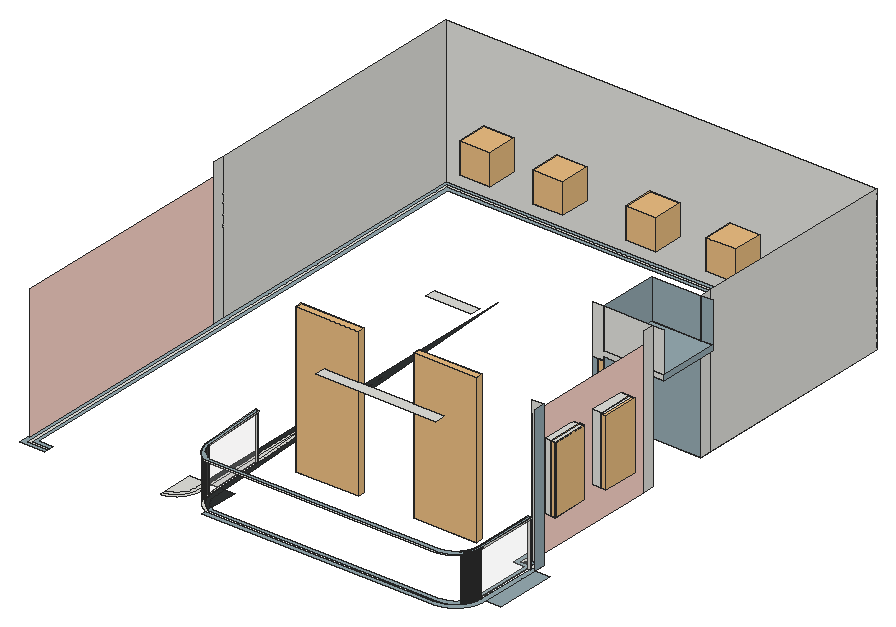
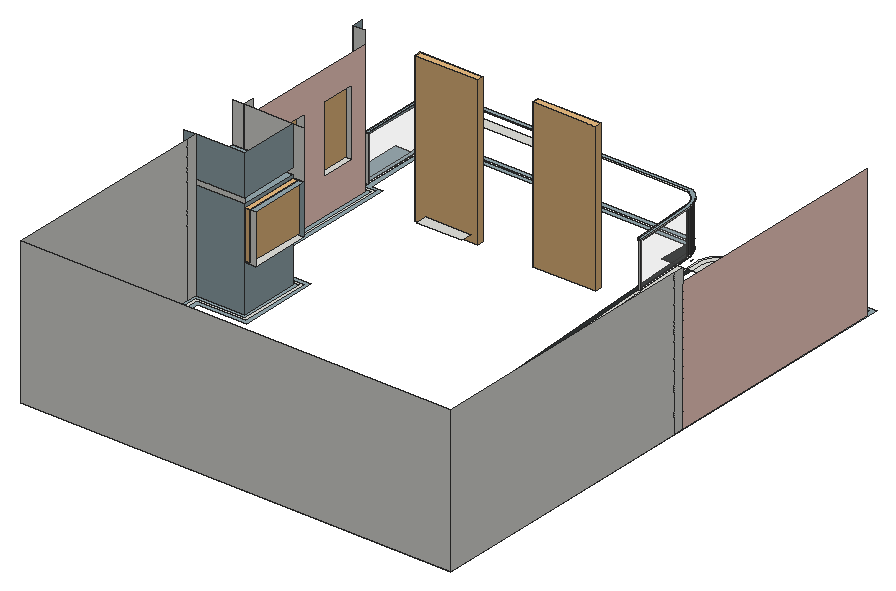
# SketchUp Ruby script. Lengths in inches.
U = 1.inch
M = Sketchup.active_model
def pt(a) = Geom::Point3d.new(a.map { |v| v * U })
def face(e, loops, mat)
  f = e.add_face(loops[0].map { |a| pt(a) })
  loops[1..].each { |l| e.add_face(l.map { |a| pt(a) }).erase! }
  f.material = f.back_material = mat if mat
  f
end
# faces: each face lists its corners as indices into pts; further lists are holes
def faces(e, pts, list, mat = nil) = list.each { |f| face(e, (f[0].is_a?(Array) ? f : [f]).map { |l| l.map { |i| pts[i] } }, mat) }
# xy, xz, yz: faces in a plane at the given z, y or x. An outline is a flat list of corners, or four numbers for a rectangle; further outlines are holes
def ring(l) = l.size == 4 ? [[l[0], l[1]], [l[2], l[1]], [l[2], l[3]], [l[0], l[3]]] : l.each_slice(2).to_a
def flat(e, list, mat, &to3) = list.each { |f| face(e, (f[0].is_a?(Array) ? f : [f]).map { |l| ring(l).map { |u, v| to3.(u, v) } }, mat) }
def xy(e, z, list, mat = nil) = flat(e, list, mat) { |x, y| [x, y, z] }
def xz(e, y, list, mat = nil) = flat(e, list, mat) { |x, z| [x, y, z] }
def yz(e, x, list, mat = nil) = flat(e, list, mat) { |y, z| [x, y, z] }
def lines(e, pts, list) = list.each { |a, b| e.add_line(pt(pts[a]), pt(pts[b])) }
# prism: a flat outline (further loops are holes) pulled along v
def prism(e, loops, v, mat = nil)
  f = face(e, loops, mat); d = Geom::Vector3d.new(v.map { |x| x * U })
  f.pushpull(f.normal.samedirection?(d) ? d.length : -d.length)
end
def box(e, o, s, mat = nil) = prism(e, [[o, [o[0] + s[0], o[1], o[2]], [o[0] + s[0], o[1] + s[1], o[2]], [o[0], o[1] + s[1], o[2]]]], [0, 0, s[2]], mat)
def at(x, y, z, deg = 0) = Geom::Transformation.translation(pt([x, y, z])) * Geom::Transformation.rotation(ORIGIN, Z_AXIS, deg.degrees)
def axes(o, x, y, z) = Geom::Transformation.new([*x, 0, *y, 0, *z, 0, *pt(o).to_a, 1])
def part(name) = M.definitions.add(name)
# library, detail: a bought-in or finely detailed component or shape, given as its bounding box
def library(name, o, s) = part(name).tap { |d| box(d.entities, o, s) }
def detail(e, o, s) = box(e.add_group.entities, o, s)
def put(e, d, t, mat = nil) = e.add_instance(d, t).tap { |i| i.material = mat if mat }
def group(e, t, mat = nil) = e.add_group.tap { |g| g.transformation = t; g.material = mat if mat }.entities
root = M.entities
M.materials.add("Generic").color = [150, 171, 178]
M.materials.add("Generic\#1").color = [47, 50, 50]
M.materials.add("Glass Thin Clear 001").color = [252, 250, 250]
M.materials["Glass Thin Clear 001"].alpha = 0.1
M.materials.add("[Color B01]").color = [255, 216, 204]
c1 = library("Curtains 003",[-24.98,-2.79,0.01],[49.96,5.58,117.31])
c2 = library("Window 46-05",[-17.86,-2.78,0],[35.72,4.26,58.96])
c3 = library("Window 46-06",[-34.91,-2.12,0],[69.82,4.27,59.06])
c4 = library("Omni Light",[-12,-12,-12],[24,24,24])
xy(root,257,[[13.326,45.171,29.81,45.171,29.81,46.928,15.083,46.928,15.083,460.197,347.352,460.197,347.352,295.928,308.352,295.928,308.352,238.197,347.352,238.197,347.352,118.197,356.352,118.197,356.352,114.0625,358.109,114.0625,358.109,119.954,349.109,119.954,349.109,239.954,310.109,239.954,310.109,294.171,349.109,294.171,349.109,461.954,13.326,461.954],[119.415,45.199,120.031,45.281,120.973,45.455,121.906,45.676,122.826,45.944,123.731,46.258,124.62,46.616,125.489,47.019,126.338,47.465,127.162,47.953,127.962,48.481,128.733,49.049,129.476,49.655,130.187,50.298,130.864,50.975,131.507,51.685,132.114,52.427,132.682,53.198,133.212,53.997,133.7,54.822,134.146,55.67,134.55,56.539,134.909,57.427,135.223,58.332,135.492,59.252,135.714,60.184,135.889,61.127,136.016,62.076,136.096,63.031,136.109,63.436,136.109,74.3125,134.352,74.3125,134.352,63.465,134.341,63.133,134.269,62.266,134.154,61.404,133.995,60.548,133.793,59.702,133.549,58.867,133.264,58.045,132.938,57.238,132.572,56.449,132.166,55.679,131.723,54.931,131.242,54.205,130.726,53.505,130.175,52.831,129.592,52.186,128.976,51.571,128.331,50.988,127.657,50.4375,126.956,49.922,126.23,49.442,125.481,48.999,124.711,48.594,123.922,48.229,123.115,47.903,122.293,47.618,121.457,47.375,120.611,47.174,119.755,47.016,119.415,46.971],[154.672,45.502,154.672,47.455,153.064,48.418,151.48,49.591,150.018,50.913,148.692,52.372,147.514,53.953,146.497,55.641,145.649,57.421,144.978,59.275,144.492,61.185,144.194,63.134,143.593,74.3125,141.834,74.3125,142.445,62.954,142.769,60.835,143.297,58.758,144.026,56.743,144.948,54.808,146.054,52.973,147.334,51.254,148.776,49.668,150.366,48.231,152.088,46.955,153.927,45.854],[119.415,46.971,119.755,47.016,120.611,47.174,121.457,47.375,122.293,47.618,123.115,47.903,123.922,48.229,124.711,48.594,125.481,48.999,126.23,49.442,126.956,49.922,127.657,50.4375,128.331,50.988,128.976,51.571,129.592,52.186,130.175,52.831,130.726,53.505,131.242,54.205,131.723,54.931,132.166,55.679,132.572,56.449,132.938,57.238,133.264,58.045,133.549,58.867,133.793,59.702,133.995,60.548,134.154,61.404,134.269,62.266,134.341,63.133,134.352,63.465,134.352,74.3125,131.151,74.3125,131.151,63.517,131.144,63.319,131.085,62.612,130.991,61.909,130.862,61.212,130.697,60.522,130.499,59.841,130.266,59.171,130,58.513,129.701,57.87,129.371,57.242,129.009,56.632,128.618,56.04,128.197,55.469,127.748,54.92,127.272,54.394,126.77,53.893,126.244,53.417,125.694,52.968,125.123,52.548,124.531,52.157,123.921,51.796,123.293,51.466,122.649,51.167,121.991,50.902,121.321,50.67,120.64,50.472,119.95,50.308,119.415,50.209],[119.415,50.209,119.95,50.308,120.64,50.472,121.321,50.67,121.991,50.902,122.649,51.167,123.293,51.466,123.921,51.796,124.531,52.157,125.123,52.548,125.694,52.968,126.244,53.417,126.77,53.893,127.272,54.394,127.748,54.92,128.197,55.469,128.618,56.04,129.009,56.632,129.371,57.242,129.701,57.87,130,58.513,130.266,59.171,130.499,59.841,130.697,60.522,130.862,61.212,130.991,61.909,131.085,62.612,131.144,63.319,131.151,63.517,131.151,74.3125,119.415,74.3125],
  [139.218,63.384,139.237,63.964,139.218,65.078],[134.352,74.3125,136.109,74.3125,136.109,180.704,139.695,114.0625,141.454,114.0625,134.352,246.036],[136.109,74.3125,141.834,74.3125,139.695,114.0625,136.109,180.704]])
xy(root,257,[[10.218,42.0625,29.81,42.0625,29.81,45.171,13.326,45.171,13.326,461.954,349.109,461.954,349.109,294.171,310.109,294.171,310.109,239.954,349.109,239.954,349.109,119.954,358.109,119.954,358.109,66.083,358.101,65.516,358.08,64.969,358.044,64.423,357.988,63.812,357.98,63.378,357.947,63.094,357.891,62.688,357.827,62.284,357.755,61.881,357.675,61.479,357.587,61.079,357.491,60.681,357.388,60.285,357.276,59.891,357.156,59.499,357.029,59.11,356.894,58.723,356.751,58.339,356.6,57.959,356.442,57.581,356.277,57.206,356.104,56.835,355.923,56.467,355.736,56.103,355.541,55.743,355.339,55.387,355.13,55.035,354.913,54.687,354.69,54.343,354.461,54.004,354.224,53.67,353.981,53.34,353.731,53.016,353.475,52.696,353.213,52.382,352.944,52.073,352.669,51.769,352.388,51.471,352.102,51.178,351.809,50.892,351.511,50.611,351.207,50.336,350.898,50.068,350.584,49.805,350.264,49.549,349.94,49.299,349.61,49.056,349.276,48.82,348.937,48.59,348.593,48.367,348.245,48.151,347.893,47.941,347.537,47.739,347.177,47.545,346.813,47.357,346.445,47.176,346.074,47.003,345.699,46.838,345.322,46.68,344.941,46.529,344.557,46.387,344.17,46.251,343.781,46.124,343.389,46.004,342.995,45.893,342.599,45.789,342.201,45.693,341.801,45.605,341.399,45.525,340.996,45.453,340.592,45.389,340.186,45.333,339.902,45.3,339.468,45.292,338.857,45.236,338.311,45.2,337.764,45.179,337.197,45.171,155.37,45.171,154.672,45.502,154.672,42.0625,337.222,42.0625,337.846,42.071,338.474,42.095,339.101,42.136,339.638,42.186,340.111,42.194,340.579,42.249,341.046,42.313,341.512,42.387,341.976,42.47,342.439,42.562,342.899,42.663,343.358,42.774,343.814,42.893,344.268,43.022,344.719,43.16,345.167,43.307,345.612,43.462,346.054,43.627,346.493,43.8,346.928,43.982,347.359,44.173,347.786,44.372,348.21,44.58,348.629,44.796,349.044,45.02,349.454,45.253,349.859,45.494,350.26,45.742,350.656,45.999,351.046,46.264,351.431,46.536,351.81,46.816,352.184,47.104,352.552,47.399,352.914,47.701,353.27,48.01,353.62,48.327,353.963,48.65,354.3,48.98,354.63,49.317,354.953,49.66,355.27,50.01,355.579,50.366,355.881,50.728,356.176,51.096,356.464,51.47,356.744,51.849,357.016,52.234,357.281,52.624,357.538,53.02,357.787,53.421,358.027,53.826,358.26,54.236,358.484,54.651,358.701,55.07,358.908,55.494,359.107,55.921,359.298,56.352,359.48,56.787,359.653,57.226,359.818,57.668,359.973,58.113,360.12,58.561,360.258,59.012,360.387,59.466,360.506,59.922,360.617,60.381,360.718,60.841,360.81,61.304,360.893,61.768,360.967,62.234,361.031,62.701,361.086,63.17,361.094,63.642,361.144,64.179,361.185,64.806,361.209,65.434,361.218,66.0625,361.218,123.0625,352.218,123.0625,352.218,243.0625,313.218,243.0625,313.218,291.0625,352.218,291.0625,352.218,465.0625,10.218,465.0625],[15.083,46.928,29.81,46.928,29.81,50.129,18.284,50.129,18.284,456.996,344.151,456.996,344.151,299.129,305.151,299.129,305.151,234.996,344.151,234.996,344.151,114.996,353.151,114.996,353.151,66.115,353.145,65.645,353.128,65.229,353.101,64.8125,353.034,64.082,353.028,63.713,352.986,63.413,352.938,63.106,352.883,62.801,352.823,62.496,352.756,62.193,352.683,61.891,352.604,61.59,352.519,61.292,352.429,60.995,352.332,60.699,352.23,60.406,352.121,60.115,352.007,59.826,351.887,59.54,351.762,59.256,351.631,58.974,351.494,58.695,351.351,58.419,351.204,58.146,351.05,57.876,350.892,57.609,350.728,57.345,350.559,57.085,350.385,56.828,350.205,56.574,350.021,56.324,349.831,56.078,349.637,55.836,349.438,55.597,349.234,55.363,349.026,55.132,348.813,54.906,348.596,54.684,348.374,54.467,348.148,54.254,347.917,54.046,347.683,53.842,347.445,53.643,347.202,53.449,346.956,53.259,346.706,53.075,346.453,52.896,346.196,52.721,345.935,52.552,345.671,52.388,345.404,52.23,345.134,52.076,344.861,51.929,344.585,51.786,344.306,51.65,344.024,51.518,343.74,51.393,343.454,51.273,343.165,51.159,342.874,51.05,342.581,50.948,342.286,50.851,341.988,50.761,341.69,50.676,341.389,50.597,341.087,50.524,340.784,50.458,340.479,50.397,340.174,50.342,339.867,50.294,339.567,50.253,339.198,50.246,338.468,50.179,338.051,50.152,337.635,50.135,337.165,50.129,156.484,50.129,156.266,50.232,154.844,51.084,154.672,51.212,154.672,47.455,154.755,47.405,155.765,46.928,337.186,46.928,337.718,46.935,338.219,46.954,338.719,46.987,339.372,47.047,339.784,47.054,339.964,47.075,340.335,47.127,340.705,47.185,341.073,47.251,341.441,47.324,341.806,47.404,342.171,47.492,342.533,47.587,342.893,47.689,343.251,47.799,343.607,47.915,343.961,48.039,344.312,48.169,344.66,48.307,345.005,48.452,345.348,48.603,345.6875,48.761,346.024,48.926,346.356,49.098,346.686,49.276,347.011,49.461,347.333,49.652,347.652,49.849,347.966,50.053,348.276,50.264,348.581,50.48,348.883,50.702,349.179,50.931,349.472,51.165,349.759,51.405,350.042,51.65,350.32,51.902,350.592,52.158,350.86,52.421,351.122,52.688,351.378,52.961,351.63,53.238,351.875,53.521,352.115,53.808,352.35,54.101,352.578,54.397,352.8,54.699,353.017,55.004,353.227,55.314,353.431,55.629,353.628,55.947,353.819,56.269,354.004,56.594,354.182,56.924,354.354,57.257,354.519,57.593,354.677,57.932,354.829,58.275,354.973,58.62,355.111,58.969,355.241,59.319,355.365,59.673,355.481,60.029,355.591,60.387,355.693,60.747,355.788,61.11,355.876,61.474,355.956,61.839,356.029,62.207,356.095,62.575,356.154,62.945,356.205,63.316,356.226,63.496,356.233,63.908,356.293,64.561,356.326,65.061,356.345,65.562,356.352,66.094,356.352,118.197,347.352,118.197,347.352,238.197,308.352,238.197,308.352,295.928,347.352,295.928,347.352,460.197,15.083,460.197],[361.218,66.0625,373.218,114.0625]],"Generic")
xy(root,257,[[154.672,47.455,154.672,51.212,153.511,52.071,152.281,53.183,151.166,54.41,150.175,55.74,149.319,57.16,148.606,58.657,148.042,60.216,147.633,61.823,147.383,63.462,146.799,74.3125,143.593,74.3125,144.194,63.134,144.492,61.185,144.978,59.275,145.649,57.421,146.497,55.641,147.514,53.953,148.692,52.372,150.018,50.913,151.48,49.591,153.064,48.418],[154.672,51.212,154.672,74.3125,146.799,74.3125,147.383,63.462,147.633,61.823,148.042,60.216,148.606,58.657,149.319,57.16,150.175,55.74,151.166,54.41,152.281,53.183,153.511,52.071],[131.151,74.3125,134.352,74.3125,134.352,246.036,141.454,114.0625,143.593,74.3125,146.799,74.3125,131.151,365.116]],"Generic\#1")
xy(root,285.591,[[352.218,135.565,361.218,163.627],[352.218,182.69,361.218,210.752]])
xy(root,293,[[155.245,44.615,153.664,45.363,151.779,46.492,150.013,47.8,148.383,49.274,146.905,50.9,145.592,52.662,144.458,54.544,143.512,56.528,142.765,58.595,142.223,60.724,141.891,62.897,139.108,114.619,141.981,114.619,144.748,63.191,145.037,61.296,145.51,59.438,146.162,57.635,146.987,55.905,147.976,54.263,149.121,52.726,150.411,51.308,151.833,50.022,153.373,48.881,155.018,47.896,155.889,47.484,337.182,47.484,337.704,47.491,338.19,47.51,338.675,47.541,339.342,47.603,339.746,47.61,339.894,47.627,340.254,47.677,340.613,47.733,340.97,47.797,341.327,47.868,341.682,47.946,342.035,48.031,342.386,48.124,342.736,48.223,343.083,48.329,343.429,48.442,343.772,48.562,344.112,48.689,344.45,48.822,344.786,48.962,345.118,49.109,345.447,49.263,345.774,49.423,346.097,49.589,346.416,49.762,346.732,49.942,347.045,50.127,347.353,50.319,347.658,50.517,347.959,50.721,348.256,50.931,348.548,51.146,348.836,51.368,349.12,51.595,349.399,51.828,349.673,52.066,349.942,52.31,350.207,52.559,350.466,52.814,350.721,53.073,350.97,53.338,351.214,53.607,351.452,53.881,351.685,54.16,351.912,54.444,352.134,54.732,352.35,55.024,352.559,55.321,352.763,55.622,352.961,55.927,353.153,56.235,353.339,56.548,353.518,56.864,353.691,57.183,353.857,57.506,354.017,57.833,354.171,58.162,354.318,58.494,354.458,58.83,354.591,59.168,354.718,59.508,354.838,59.851,354.951,60.197,355.057,60.544,355.157,60.894,355.249,61.245,355.334,61.599,355.412,61.953,355.483,62.31,355.547,62.668,355.604,63.026,355.653,63.386,355.67,63.534,355.677,63.938,355.739,64.605,355.77,65.09,355.79,65.576,355.796,66.098,355.796,114.619,358.665,114.619,358.665,66.079,358.657,65.501,358.635,64.94,358.599,64.38,358.544,63.781,358.536,63.341,358.499,63.024,358.441,62.607,358.376,62.192,358.302,61.778,358.22,61.365,358.129,60.954,358.031,60.545,357.924,60.138,357.809,59.734,357.686,59.331,357.555,58.932,357.417,58.535,357.27,58.14,357.115,57.749,356.953,57.361,356.783,56.976,356.605,56.595,356.42,56.217,356.227,55.843,356.027,55.474,355.82,55.108,355.605,54.746,355.383,54.389,355.154,54.036,354.918,53.6875,354.675,53.344,354.425,53.006,354.169,52.672,353.905,52.344,353.636,52.021,353.36,51.704,353.078,51.392,352.789,51.086,352.495,50.785,352.194,50.491,351.888,50.202,351.576,49.92,351.259,49.644,350.936,49.375,350.608,49.112,350.274,48.855,349.936,48.605,349.592,48.362,349.244,48.126,348.891,47.897,348.534,47.675,348.172,47.461,347.807,47.253,347.437,47.053,347.063,46.86,346.685,46.675,346.304,46.497,345.919,46.327,345.531,46.165,345.14,46.01,344.746,45.863,344.348,45.725,343.949,45.594,343.546,45.471,343.142,45.356,342.735,45.249,342.326,45.151,341.915,45.06,341.503,44.978,341.088,44.904,340.673,44.839,340.256,44.781,339.939,44.744,339.499,44.736,338.9,44.681,338.34,44.645,337.779,44.623,337.201,44.615]])
xy(root,294,[[155.245,44.615,337.201,44.615,337.779,44.623,338.34,44.645,338.9,44.681,339.499,44.736,339.939,44.744,340.256,44.781,340.673,44.839,341.088,44.904,341.503,44.978,341.915,45.06,342.326,45.151,342.735,45.249,343.142,45.356,343.546,45.471,343.949,45.594,344.348,45.725,344.746,45.863,345.14,46.01,345.531,46.165,345.919,46.327,346.304,46.497,346.685,46.675,347.063,46.86,347.437,47.053,347.807,47.253,348.172,47.461,348.534,47.675,348.891,47.897,349.244,48.126,349.592,48.362,349.936,48.605,350.274,48.855,350.608,49.112,350.936,49.375,351.259,49.644,351.576,49.92,351.888,50.202,352.194,50.491,352.495,50.785,352.789,51.086,353.078,51.392,353.36,51.704,353.636,52.021,353.905,52.344,354.169,52.672,354.425,53.006,354.675,53.344,354.918,53.6875,355.154,54.036,355.383,54.389,355.605,54.746,355.82,55.108,356.027,55.474,356.227,55.843,356.42,56.217,356.605,56.595,356.783,56.976,356.953,57.361,357.115,57.749,357.27,58.14,357.417,58.535,357.555,58.932,357.686,59.331,357.809,59.734,357.924,60.138,358.031,60.545,358.129,60.954,358.22,61.365,358.302,61.778,358.376,62.192,358.441,62.607,358.499,63.024,358.536,63.341,358.544,63.781,358.599,64.38,358.635,64.94,358.657,65.501,358.665,66.079,358.665,114.619,355.796,114.619,355.796,66.098,355.79,65.576,355.77,65.09,355.739,64.605,355.677,63.938,355.67,63.534,355.653,63.386,355.604,63.026,355.547,62.668,355.483,62.31,355.412,61.953,355.334,61.599,355.249,61.245,355.157,60.894,355.057,60.544,354.951,60.197,354.838,59.851,354.718,59.508,354.591,59.168,354.458,58.83,354.318,58.494,354.171,58.162,354.017,57.833,353.857,57.506,353.691,57.183,353.518,56.864,353.339,56.548,353.153,56.235,352.961,55.927,352.763,55.622,352.559,55.321,352.35,55.024,352.134,54.732,351.912,54.444,351.685,54.16,351.452,53.881,351.214,53.607,350.97,53.338,350.721,53.073,350.466,52.814,350.207,52.559,349.942,52.31,349.673,52.066,349.399,51.828,349.12,51.595,348.836,51.368,348.548,51.146,348.256,50.931,347.959,50.721,347.658,50.517,347.353,50.319,347.045,50.127,346.732,49.942,346.416,49.762,346.097,49.589,345.774,49.423,345.447,49.263,345.118,49.109,344.786,48.962,344.45,48.822,344.112,48.689,343.772,48.562,343.429,48.442,343.083,48.329,342.736,48.223,342.386,48.124,342.035,48.031,341.682,47.946,341.327,47.868,340.97,47.797,340.613,47.733,340.254,47.677,339.894,47.627,339.746,47.61,339.342,47.603,338.675,47.541,338.19,47.51,337.704,47.491,337.182,47.484,155.889,47.484,155.018,47.896,153.373,48.881,151.833,50.022,150.411,51.308,149.121,52.726,147.976,54.263,146.987,55.905,146.162,57.635,145.51,59.438,145.037,61.296,144.748,63.191,141.981,114.619,139.108,114.619,141.891,62.897,142.223,60.724,142.765,58.595,143.512,56.528,144.458,54.544,145.592,52.662,146.905,50.9,148.383,49.274,150.013,47.8,151.779,46.492,153.664,45.363]],"Generic")
xy(root,294.452,[[304.218,243.0625,313.218,291.0625]])
xy(root,333.326,[[304.218,243.0625,313.218,291.0625]],"Generic")
xy(root,335.818,[[313.218,243.0625,361.218,291.0625]],"Generic")
xy(root,336,[[187.218,114.0625,283.218,123.0625],[179.03,234.0625,215.03,243.0625]])
xy(root,338.859,[[352.218,135.565,361.218,163.627],[352.218,182.69,361.218,210.752]])
xy(root,340.246,[[313.218,243.0625,361.218,291.0625]],"Generic")
xz(root,114.0625,[[139.695,257,141.454,293],[356.352,257,358.109,293]])
xz(root,114.619,[[139.108,293,141.981,294],[355.796,293,358.665,294]])
xz(root,123.0625,[[352.218,257,361.218,372]])
xz(root,135.565,[[352.218,285.591,361.218,338.859]])
xz(root,163.627,[[352.218,285.591,361.218,338.859]])
xz(root,182.69,[[352.218,285.591,361.218,338.859]])
xz(root,210.752,[[352.218,285.591,361.218,338.859]])
xz(root,243.0625,[[304.218,333.326,304.218,372,313.218,372,313.218,340.246,352.218,340.246,352.218,335.818,313.218,335.818,313.218,333.326],[352.218,335.818,361.218,340.246],[313.218,340.246,352.218,372],[352.218,340.246,361.218,372]])
xz(root,243.0625,[[313.218,257,313.218,294.452,304.218,294.452,304.218,333.326,313.218,333.326,313.218,335.818,352.218,335.818,352.218,257]],"Generic")
xz(root,291.0625,[[304.218,294.452,313.218,333.326],[313.218,335.818,352.218,340.246],[352.218,335.818,361.218,340.246]])
xz(root,291.0625,[[313.218,257,352.218,335.818],[313.218,340.246,352.218,372],[352.218,340.246,361.218,372]],"Generic")
xz(root,465.0625,[[10.218,257,352.218,372]])
yz(root,10.218,[[234.0625,257,243.0625,372],[243.0625,257,465.0625,372]])
yz(root,10.218,[[51.0625,257,234.0625,362]],"[Color B01]")
yz(root,313.218,[[243.0625,257,291.0625,294.452],[243.0625,333.326,291.0625,335.818],[243.0625,340.246,291.0625,372]],"Generic")
yz(root,352.218,[[234.0625,257,243.0625,372],[291.0625,257,300.0625,372],[300.0625,257,465.0625,372]])
yz(root,352.218,[[[123.0625,257,234.0625,362],[182.69,285.591,210.752,338.859],[135.565,285.591,163.627,338.859]]],"[Color B01]")
yz(root,355.796,[[114.0625,293,114.619,294]])
yz(root,355.796,[[66.098,293,114.0625,294]],"Generic")
yz(root,355.977,[[66.097,293,111.931,294]])
yz(root,356.352,[[66.094,257,114.0625,293]],"Glass Thin Clear 001")
yz(root,358.109,[[66.083,257,114.0625,293]],"Glass Thin Clear 001")
yz(root,358.484,[[66.08,293,111.931,294]])
yz(root,358.665,[[66.079,293,114.619,294]])
yz(root,361.218,[[114.0625,257,123.0625,372],[243.0625,335.818,291.0625,340.246]],"Generic")
p = [[148.692,52.372,257],[147.514,53.953,257],[147.514,53.953,293],[148.692,52.372,293],[144.948,54.808,257],[146.054,52.973,257],
  [146.054,52.973,293],[144.948,54.808,293],[351.63,53.238,257],[351.378,52.961,257],[351.378,52.961,293],[351.63,53.238,293],
  [353.731,53.016,257],[353.981,53.34,257],[353.981,53.34,293],[353.731,53.016,293],[351.875,53.521,257],[351.875,53.521,293],
  [354.224,53.67,257],[354.224,53.67,293],[352.115,53.808,257],[352.115,53.808,293],[354.461,54.004,257],[354.461,54.004,293],
  [352.35,54.101,257],[352.35,54.101,293],[146.497,55.641,257],[146.497,55.641,293],[354.69,54.343,257],[354.69,54.343,293],
  [352.578,54.397,257],[352.578,54.397,293],[354.913,54.687,257],[354.913,54.687,293],[352.8,54.699,257],[352.8,54.699,293],
  [353.017,55.004,257],[353.017,55.004,293],[355.13,55.035,257],[355.13,55.035,293],[144.026,56.743,257],[144.026,56.743,293],
  [353.227,55.314,257],[353.227,55.314,293],[355.339,55.387,257],[355.339,55.387,293],[353.431,55.629,257],[353.431,55.629,293],
  [355.541,55.743,257],[355.541,55.743,293],[145.649,57.421,257],[145.649,57.421,293],[353.628,55.947,257],[353.628,55.947,293],
  [355.736,56.103,257],[355.736,56.103,293],[353.819,56.269,257],[353.819,56.269,293],[355.923,56.467,257],[355.923,56.467,293],
  [354.004,56.594,257],[354.004,56.594,293],[356.104,56.835,257],[356.104,56.835,293],[354.182,56.924,257],[354.182,56.924,293],
  [143.297,58.758,257],[143.297,58.758,293],[356.277,57.206,257],[356.277,57.206,293],[354.354,57.257,257],[354.354,57.257,293],
  [356.442,57.581,257],[356.442,57.581,293],[354.519,57.593,257],[354.519,57.593,293],[144.978,59.275,257],[144.978,59.275,293],
  [354.677,57.932,257],[354.677,57.932,293],[356.6,57.959,257],[356.6,57.959,293],[354.829,58.275,257],[354.829,58.275,293],
  [356.751,58.339,257],[356.751,58.339,293],[354.973,58.62,257],[354.973,58.62,293],[356.894,58.723,257],[356.894,58.723,293],
  [355.111,58.969,257],[355.111,58.969,293],[357.029,59.11,257],[357.029,59.11,293],[142.769,60.835,257],[142.769,60.835,293],
  [355.241,59.319,257],[355.241,59.319,293],[357.156,59.499,257],[357.156,59.499,293],[144.492,61.185,257],[144.492,61.185,293],
  [355.365,59.673,257],[355.365,59.673,293],[357.276,59.891,257],[357.276,59.891,293],[355.481,60.029,257],[355.481,60.029,293],
  [357.388,60.285,257],[357.388,60.285,293],[355.591,60.387,257],[355.591,60.387,293],[357.491,60.681,257],[357.491,60.681,293],
  [355.693,60.747,257],[355.693,60.747,293],[355.788,61.11,257],[355.788,61.11,293],[357.587,61.079,257],[357.587,61.079,293],
  [142.445,62.954,257],[142.445,62.954,293],[355.876,61.474,257],[355.876,61.474,293],[357.675,61.479,257],[357.675,61.479,293],
  [144.194,63.134,257],[144.194,63.134,293],[355.956,61.839,257],[355.956,61.839,293],[357.755,61.881,257],[357.755,61.881,293],
  [356.029,62.207,257],[356.029,62.207,293],[357.827,62.284,257],[357.827,62.284,293],[356.095,62.575,257],[356.095,62.575,293],
  [357.891,62.688,257],[357.891,62.688,293],[356.154,62.945,257],[356.154,62.945,293],[357.947,63.094,257],[357.947,63.094,293],
  [356.205,63.316,257],[356.205,63.316,293],[139.695,114.0625,257],[141.834,74.3125,257],[139.695,114.0625,293],[143.593,74.3125,257],
  [141.454,114.0625,257],[141.454,114.0625,293],[357.98,63.378,257],[357.98,63.378,293],[356.226,63.496,257],[356.226,63.496,293],
  [357.988,63.812,257],[357.988,63.812,293],[356.233,63.908,257],[356.233,63.908,293],[358.044,64.423,257],[358.044,64.423,293],
  [356.293,64.561,257],[356.293,64.561,293],[358.08,64.969,257],[358.08,64.969,293],[356.326,65.061,257],[356.326,65.061,293],
  [358.101,65.516,257],[358.101,65.516,293],[356.345,65.562,257],[356.345,65.562,293],[358.109,66.083,257],[358.109,66.083,293],
  [356.352,66.094,257],[356.352,66.094,293],[147.826,54.162,293],[147.826,54.162,294],[148.982,52.611,294],[148.982,52.611,293],
  [144.458,54.544,294],[144.458,54.544,293],[145.592,52.662,293],[145.592,52.662,294],[149.121,52.726,294],[149.121,52.726,293],
  [147.976,54.263,293],[147.976,54.263,294],[145.742,52.763,293],[145.742,52.763,294],[144.617,54.63,294],[144.617,54.63,293],
  [350.851,52.948,293],[350.851,52.948,294],[351.103,53.215,294],[351.103,53.215,293],[354.425,53.006,294],[354.425,53.006,293],
  [354.675,53.344,293],[354.675,53.344,294],[350.97,53.338,294],[350.97,53.338,293],[350.721,53.073,293],[350.721,53.073,294],
  [354.528,53.45,293],[354.528,53.45,294],[354.28,53.115,294],[354.28,53.115,293],[351.349,53.487,294],[351.349,53.487,293],
  [351.214,53.607,294],[351.214,53.607,293],[354.918,53.6875,293],[354.918,53.6875,294],[351.59,53.764,294],[351.59,53.764,293],
  [354.769,53.791,293],[354.769,53.791,294],[351.452,53.881,294],[351.452,53.881,293],[355.154,54.036,293],[355.154,54.036,294],
  [351.825,54.046,294],[351.825,54.046,293],[355.003,54.136,293],[355.003,54.136,294],[351.685,54.16,294],[351.685,54.16,293],
  [352.055,54.332,294],[352.055,54.332,293],[355.383,54.389,293],[355.383,54.389,294],[355.23,54.486,293],[355.23,54.486,294],
  [146.827,55.819,293],[146.827,55.819,294],[351.912,54.444,294],[351.912,54.444,293],[146.987,55.905,293],[146.987,55.905,294],
  [352.278,54.623,294],[352.278,54.623,293],[352.134,54.732,294],[352.134,54.732,293],[355.605,54.746,293],[355.605,54.746,294],
  [143.512,56.528,294],[143.512,56.528,293],[355.45,54.84,293],[355.45,54.84,294],[143.679,56.598,294],[143.679,56.598,293],
  [352.496,54.918,294],[352.496,54.918,293],[352.35,55.024,294],[352.35,55.024,293],[355.82,55.108,293],[355.82,55.108,294],
  [355.663,55.199,293],[355.663,55.199,294],[352.708,55.218,294],[352.708,55.218,293],[352.559,55.321,294],[352.559,55.321,293],
  [356.027,55.474,293],[356.027,55.474,294],[352.914,55.522,294],[352.914,55.522,293],[355.869,55.561,293],[355.869,55.561,294],
  [352.763,55.622,294],[352.763,55.622,293],[353.114,55.83,294],[353.114,55.83,293],[356.227,55.843,293],[356.227,55.843,294],
  [352.961,55.927,294],[352.961,55.927,293],[356.067,55.928,293],[356.067,55.928,294],[145.995,57.566,293],[145.995,57.566,294],
  [353.308,56.141,294],[353.308,56.141,293],[356.42,56.217,293],[356.42,56.217,294],[146.162,57.635,293],[146.162,57.635,294],
  [353.153,56.235,294],[353.153,56.235,293],[356.258,56.299,293],[356.258,56.299,294],[353.495,56.457,294],[353.495,56.457,293],
  [353.339,56.548,294],[353.339,56.548,293],[356.605,56.595,293],[356.605,56.595,294],[356.442,56.673,293],[356.442,56.673,294],
  [142.765,58.595,294],[142.765,58.595,293],[353.518,56.864,294],[353.518,56.864,293],[353.676,56.776,294],[353.676,56.776,293],
  [142.938,58.648,294],[142.938,58.648,293],[356.783,56.976,293],[356.783,56.976,294],[356.618,57.051,293],[356.618,57.051,294],
  [353.851,57.099,294],[353.851,57.099,293],[353.691,57.183,294],[353.691,57.183,293],[356.953,57.361,293],[356.953,57.361,294],
  [354.019,57.425,294],[354.019,57.425,293],[356.787,57.433,293],[356.787,57.433,294],[353.857,57.506,294],[353.857,57.506,293],
  [354.181,57.755,294],[354.181,57.755,293],[356.948,57.817,293],[356.948,57.817,294],[357.115,57.749,293],[357.115,57.749,294],
  [354.017,57.833,294],[354.017,57.833,293],[145.337,59.385,293],[145.337,59.385,294],[145.51,59.438,293],[145.51,59.438,294],
  [357.27,58.14,293],[357.27,58.14,294],[354.171,58.162,294],[354.171,58.162,293],[354.336,58.087,294],[354.336,58.087,293],
  [357.101,58.205,293],[357.101,58.205,294],[354.484,58.423,294],[354.484,58.423,293],[357.417,58.535,293],[357.417,58.535,294],
  [354.318,58.494,294],[354.318,58.494,293],[357.246,58.596,293],[357.246,58.596,294],[354.626,58.761,294],[354.626,58.761,293],
  [354.458,58.83,294],[354.458,58.83,293],[357.555,58.932,293],[357.555,58.932,294],[142.223,60.724,294],[142.223,60.724,293],
  [142.401,60.76,294],[142.401,60.76,293],[357.384,58.99,293],[357.384,58.99,294],[354.591,59.168,294],[354.591,59.168,293],
  [354.761,59.103,294],[354.761,59.103,293],[357.686,59.331,293],[357.686,59.331,294],[357.514,59.386,293],[357.514,59.386,294],
  [354.889,59.447,294],[354.889,59.447,293],[354.718,59.508,294],[354.718,59.508,293],[357.809,59.734,293],[357.809,59.734,294],
  [144.86,61.26,293],[144.86,61.26,294],[145.037,61.296,293],[145.037,61.296,294],[355.01,59.793,294],[355.01,59.793,293],
  [357.636,59.785,293],[357.636,59.785,294],[354.838,59.851,294],[354.838,59.851,293],[357.924,60.138,293],[357.924,60.138,294],
  [355.124,60.142,294],[355.124,60.142,293],[357.749,60.186,293],[357.749,60.186,294],[354.951,60.197,294],[354.951,60.197,293],
  [355.231,60.493,294],[355.231,60.493,293],[358.031,60.545,293],[358.031,60.545,294],[355.057,60.544,294],[355.057,60.544,293],
  [357.855,60.589,293],[357.855,60.589,294],[355.157,60.894,294],[355.157,60.894,293],[355.331,60.846,294],[355.331,60.846,293],
  [358.129,60.954,293],[358.129,60.954,294],[357.953,60.995,293],[357.953,60.995,294],[141.891,62.897,294],[141.891,62.897,293],
  [142.072,62.915,294],[142.072,62.915,293],[355.424,61.201,294],[355.424,61.201,293],[355.249,61.245,294],[355.249,61.245,293],
  [358.042,61.402,293],[358.042,61.402,294],[358.22,61.365,293],[358.22,61.365,294],[355.334,61.599,294],[355.334,61.599,293],
  [355.51,61.558,294],[355.51,61.558,293],[144.568,63.172,293],[144.568,63.172,294],[144.748,63.191,293],[144.748,63.191,294],
  [358.124,61.811,293],[358.124,61.811,294],[358.302,61.778,293],[358.302,61.778,294],[355.412,61.953,294],[355.412,61.953,293],
  [355.589,61.916,294],[355.589,61.916,293],[358.197,62.222,293],[358.197,62.222,294],[358.376,62.192,293],[358.376,62.192,294],
  [355.661,62.276,294],[355.661,62.276,293],[355.483,62.31,294],[355.483,62.31,293],[358.262,62.634,293],[358.262,62.634,294],
  [358.441,62.607,293],[358.441,62.607,294],[355.547,62.668,294],[355.547,62.668,293],[355.725,62.637,294],[355.725,62.637,293],
  [355.783,63,294],[355.783,63,293],[358.319,63.047,293],[358.319,63.047,294],[358.499,63.024,293],[358.499,63.024,294],
  [355.604,63.026,294],[355.604,63.026,293],[139.108,114.619,294],[139.108,114.619,293],[139.434,111.931,294],[139.434,111.931,293],
  [355.653,63.386,294],[355.653,63.386,293],[355.833,63.364,294],[355.833,63.364,293],[358.355,63.353,293],[358.355,63.353,294],
  [358.536,63.341,293],[358.536,63.341,294],[141.944,111.931,293],[141.944,111.931,294],[141.981,114.619,293],[141.981,114.619,294],
  [358.544,63.781,293],[358.544,63.781,294],[355.67,63.534,294],[355.67,63.534,293],[355.851,63.522,294],[355.851,63.522,293],
  [358.363,63.791,293],[358.363,63.791,294],[355.677,63.938,294],[355.677,63.938,293],[355.858,63.928,294],[355.858,63.928,293],
  [358.418,64.394,293],[358.418,64.394,294],[358.599,64.38,293],[358.599,64.38,294],[355.739,64.605,294],[355.739,64.605,293],
  [355.919,64.591,294],[355.919,64.591,293],[358.455,64.95,293],[358.455,64.95,294],[358.635,64.94,293],[358.635,64.94,294],
  [355.77,65.09,294],[355.77,65.09,293],[355.951,65.081,294],[355.951,65.081,293],[358.476,65.506,293],[358.476,65.506,294],
  [358.657,65.501,293],[358.657,65.501,294],[355.79,65.576,294],[355.79,65.576,293],[355.971,65.571,294],[355.971,65.571,293],
  [358.484,66.08,293],[358.484,66.08,294],[358.665,66.079,293],[358.665,66.079,294],[355.796,66.098,294],[355.796,66.098,293],
  [355.977,66.097,294],[355.977,66.097,293]]
faces(root,p,[[0,1,2,3],[4,5,6,7],[8,9,10,11],[12,13,14,15],[16,8,11,17],[13,18,19,14],[20,16,17,21],[18,22,23,19],
  [24,20,21,25],[1,26,27,2],[22,28,29,23],[30,24,25,31],[28,32,33,29],[34,30,31,35],[36,34,35,37],[32,38,39,33],
  [40,4,7,41],[42,36,37,43],[38,44,45,39],[46,42,43,47],[44,48,49,45],[26,50,51,27],[52,46,47,53],[48,54,55,49],
  [56,52,53,57],[54,58,59,55],[60,56,57,61],[58,62,63,59],[64,60,61,65],[66,40,41,67],[62,68,69,63],[70,64,65,71],
  [68,72,73,69],[74,70,71,75],[50,76,77,51],[78,74,75,79],[72,80,81,73],[82,78,79,83],[80,84,85,81],[86,82,83,87],
  [84,88,89,85],[90,86,87,91],[88,92,93,89],[94,66,67,95],[96,90,91,97],[92,98,99,93],[76,100,101,77],[102,96,97,103],
  [98,104,105,99],[106,102,103,107],[104,108,109,105],[110,106,107,111],[108,112,113,109],[114,110,111,115],[116,114,115,117],[112,118,119,113],
  [120,94,95,121],[122,116,117,123],[118,124,125,119],[100,126,127,101],[128,122,123,129],[124,130,131,125],[132,128,129,133],[130,134,135,131],
  [136,132,133,137],[134,138,139,135],[140,136,137,141],[138,142,143,139],[144,140,141,145],[146,147,120,121,148],[149,150,151,127,126],[142,152,153,143],
  [154,144,145,155],[152,156,157,153],[158,154,155,159],[156,160,161,157],[162,158,159,163],[160,164,165,161],[166,162,163,167],[164,168,169,165],
  [170,166,167,171],[168,172,173,169],[174,170,171,175]],"Glass Thin Clear 001")
faces(root,p,[[176,177,178,179],[180,181,182,183],[184,185,186,187],[188,189,190,191],[192,193,194,195],[196,197,198,199],[200,201,202,203],[204,205,206,207],
  [195,194,208,209],[210,211,201,200],[199,198,212,213],[209,208,214,215],[216,217,205,204],[213,212,220,221],[215,214,222,223],[224,225,217,216],
  [226,227,219,218],[223,222,228,229],[221,220,230,231],[232,233,225,224],[234,235,177,176],[187,186,238,239],[229,228,240,241],[231,230,244,245],
  [246,247,181,180],[248,249,233,232],[191,190,250,251],[241,240,252,253],[245,244,256,257],[258,259,249,248],[253,252,260,261],[257,256,264,265],
  [261,260,266,267],[268,269,259,258],[267,266,272,273],[265,264,274,275],[278,279,269,268],[280,281,235,234],[273,272,282,283],[275,274,284,285],
  [239,238,286,287],[290,291,279,278],[283,282,292,293],[285,284,296,297],[298,299,291,290],[300,301,247,246],[293,292,304,305],[251,250,306,307],
  [297,296,308,309],[310,311,299,298],[305,304,312,313],[309,308,316,317],[313,312,318,319],[320,321,311,310],[319,318,324,325],[326,327,321,320],
  [317,316,328,329],[332,333,281,280],[287,286,334,335],[329,328,336,337],[325,324,340,341],[342,343,327,326],[341,340,344,345],[337,336,346,347],
  [350,351,343,342],[345,344,352,353],[347,346,356,357],[358,359,301,300],[307,306,360,361],[362,363,351,350],[353,352,366,367],[357,356,368,369],
  [370,371,363,362],[367,366,372,373],[369,368,376,377],[378,379,333,332],[335,334,380,381],[373,372,382,383],[384,385,371,370],[377,376,388,389],
  [383,382,390,391],[392,393,385,384],[391,390,396,397],[389,388,398,399],[402,403,393,392],[397,396,406,407],[399,398,408,409],[410,411,403,402],
  [412,413,359,358],[361,360,414,415],[407,406,416,417],[420,421,411,410],[409,408,422,423],[417,416,426,427],[428,429,379,378],[381,380,430,431],
  [432,433,421,420],[423,422,434,435],[427,426,438,439],[440,441,433,432],[435,434,442,443],[439,438,444,445],[448,449,441,440],[443,442,450,451],
  [445,444,454,455],[455,454,456,457],[458,459,449,448],[451,450,460,461],[464,465,413,412],[415,414,466,467],[457,456,470,471],[472,473,459,458],
  [461,460,474,475],[476,477,429,428],[431,430,478,479],[475,474,480,481],[471,470,484,485],[486,487,473,472],[485,484,490,491],[492,493,487,486],
  [481,480,494,495],[491,490,498,499],[500,501,493,492],[495,494,502,503],[499,498,506,507],[508,509,501,500],[503,502,510,511],[507,506,514,515],
  [516,517,509,508],[511,510,518,519],[515,514,522,523]])
faces(root,p,[[218,219,211,210],[236,237,227,226],[242,243,237,236],[254,255,243,242],[262,263,255,254],[270,271,263,262],[276,277,271,270],[288,289,277,276],
  [294,295,289,288],[302,303,295,294],[314,315,303,302],[322,323,315,314],[330,331,323,322],[338,339,331,330],[348,349,339,338],[354,355,349,348],
  [364,365,355,354],[374,375,365,364],[386,387,375,374],[394,395,387,386],[400,401,395,394],[404,405,401,400],[418,419,405,404],[424,425,419,418],
  [436,437,425,424],[446,447,437,436],[452,453,447,446],[462,463,453,452],[468,469,463,462],[482,483,469,468],[488,489,483,482],[496,497,489,488],
  [504,505,497,496],[512,513,505,504],[520,521,513,512]],"Generic")
put(root,c1,at(189.17,125.86,254.68))
put(root,c1,at(282.92,125.86,254.68))
put(root,c2,axes([358.39,149.9,285.54],[0,0.80542,0],[-0.8,0,0],[0,0,0.90212]))
put(root,c2,axes([360.98,196.22,285.47],[0,0.78717,0],[-1,0,0],[0,0,0.90321]))
put(root,c3,axes([311.02,267,295.18],[0,0.68932,0],[-1.0371,0,0],[0,0,0.64598]))
put(root,c4,at(114.47,448.09,298.5))
put(root,c4,at(188.35,448.09,298.5))
put(root,c4,at(56.1,448.09,298.5))
put(root,c4,at(251.97,448.09,298.5))
